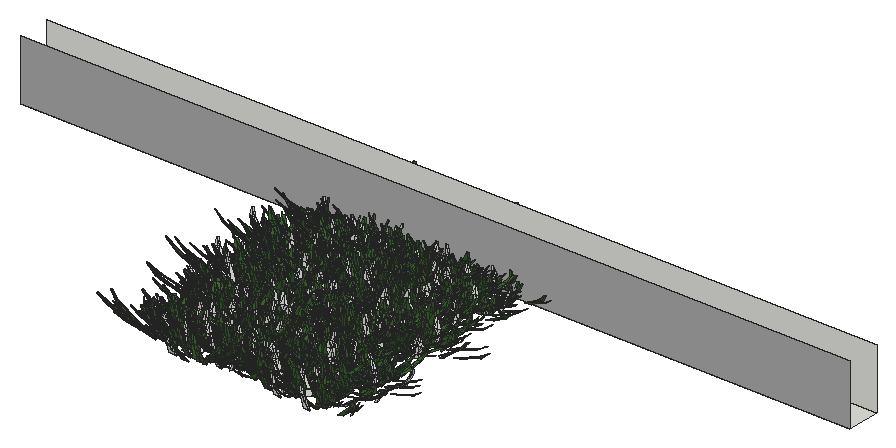
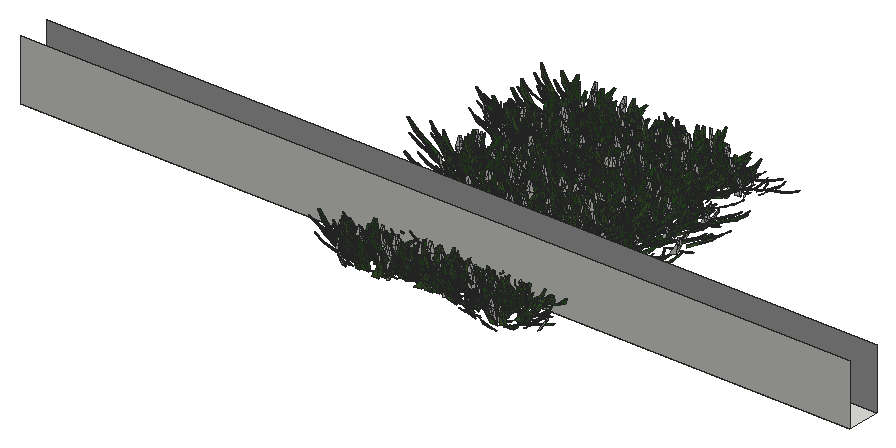
# SketchUp Ruby script. Lengths in inches.
U = 1.inch
M = Sketchup.active_model
def pt(a) = Geom::Point3d.new(a.map { |v| v * U })
def face(e, loops, mat)
  f = e.add_face(loops[0].map { |a| pt(a) })
  loops[1..].each { |l| e.add_face(l.map { |a| pt(a) }).erase! }
  f.material = f.back_material = mat if mat
  f
end
# faces: each face lists its corners as indices into pts; further lists are holes
def faces(e, pts, list, mat = nil) = list.each { |f| face(e, (f[0].is_a?(Array) ? f : [f]).map { |l| l.map { |i| pts[i] } }, mat) }
# xy, xz, yz: faces in a plane at the given z, y or x. An outline is a flat list of corners, or four numbers for a rectangle; further outlines are holes
def ring(l) = l.size == 4 ? [[l[0], l[1]], [l[2], l[1]], [l[2], l[3]], [l[0], l[3]]] : l.each_slice(2).to_a
def flat(e, list, mat, &to3) = list.each { |f| face(e, (f[0].is_a?(Array) ? f : [f]).map { |l| ring(l).map { |u, v| to3.(u, v) } }, mat) }
def xy(e, z, list, mat = nil) = flat(e, list, mat) { |x, y| [x, y, z] }
def xz(e, y, list, mat = nil) = flat(e, list, mat) { |x, z| [x, y, z] }
def yz(e, x, list, mat = nil) = flat(e, list, mat) { |y, z| [x, y, z] }
def lines(e, pts, list) = list.each { |a, b| e.add_line(pt(pts[a]), pt(pts[b])) }
# prism: a flat outline (further loops are holes) pulled along v
def prism(e, loops, v, mat = nil)
  f = face(e, loops, mat); d = Geom::Vector3d.new(v.map { |x| x * U })
  f.pushpull(f.normal.samedirection?(d) ? d.length : -d.length)
end
def box(e, o, s, mat = nil) = prism(e, [[o, [o[0] + s[0], o[1], o[2]], [o[0] + s[0], o[1] + s[1], o[2]], [o[0], o[1] + s[1], o[2]]]], [0, 0, s[2]], mat)
def at(x, y, z, deg = 0) = Geom::Transformation.translation(pt([x, y, z])) * Geom::Transformation.rotation(ORIGIN, Z_AXIS, deg.degrees)
def axes(o, x, y, z) = Geom::Transformation.new([*x, 0, *y, 0, *z, 0, *pt(o).to_a, 1])
def part(name) = M.definitions.add(name)
# library, detail: a bought-in or finely detailed component or shape, given as its bounding box
def library(name, o, s) = part(name).tap { |d| box(d.entities, o, s) }
def detail(e, o, s) = box(e.add_group.entities, o, s)
def put(e, d, t, mat = nil) = e.add_instance(d, t).tap { |i| i.material = mat if mat }
def group(e, t, mat = nil) = e.add_group.tap { |g| g.transformation = t; g.material = mat if mat }.entities
root = M.entities
M.materials.add("Material82").color = [68, 110, 58]
M.materials.add("Material83").color = [48, 90, 38]
M.materials.add("Material84").color = [68, 110, 48]
M.materials.add("Material85").color = [48, 90, 48]
M.materials.add("Material86").color = [58, 110, 58]
M.materials.add("Material87").color = [58, 90, 38]
M.materials.add("Material88").color = [68, 100, 58]
M.materials.add("Material89").color = [48, 100, 38]
M.materials.add("[Color M03]1").color = [170, 170, 170]
c1 = part("grass00")
p = [[-0.6875,0.15,0],[-0.56,0.08,5.52],[-0.04,0.03,2.76],[0.48,-0.02,0],[0.35,-0.02,5.52],[-0.1,-0.14,5.52],
  [-0.12,0.65,8.37],[-0.42,0.65,8.37]]
faces(c1.entities,p,[[0,1,2,3],[3,2,4],[1,5,2],[5,4,2],[1,6,5],[4,5,6],[7,6,1]])
c2 = part("Group16\#1")
put(c2.entities,c1,axes([1.44,-0.61,-0.01],[0.05352,0.12609,0],[-0.10704,0.04543,0.07239],[0.06664,-0.02828,0.11628]),"Material85")
put(c2.entities,c1,axes([0.76,-0.15,-0.01],[0.04676,0.24062,0],[-0.23162,0.04501,0.06642],[0.0652,-0.01267,0.23595]),"Material82")
put(c2.entities,c1,axes([0.79,0.01,-0.01],[-0.00606,0.34651,0],[-0.34381,-0.00602,0.0432],[0.04319,0.00076,0.34386]))
put(c2.entities,c1,axes([1,0.23,-0.01],[-0.07192,0.31144,0],[-0.28722,-0.06632,0.1236],[0.12043,0.02781,0.29478]),"Material84")
put(c2.entities,c1,axes([1.66,0.77,-0.01],[-0.13828,0.29651,0],[-0.21551,-0.1005,0.22471],[0.20365,0.09498,0.23779]),"Material89")
put(c2.entities,c1,axes([0.6875,0.52,-0.01],[-0.18126,0.24051,0],[-0.22746,-0.17142,0.09788],[0.07817,0.05891,0.28481]),"Material84")
put(c2.entities,c1,axes([0.68,0.78,-0.01],[-0.215,0.18688,0],[-0.12385,-0.14248,0.21334],[0.13995,0.16101,0.18878]),"Material82")
put(c2.entities,c1,axes([0.56,1,-0.01],[-0.13756,0.07624,0],[-0.06159,-0.11112,0.0927],[0.04494,0.08108,0.12705]),"Material84")
put(c2.entities,c1,axes([0.2,0.64,-0.01],[-0.23729,0.07254,0],[-0.05711,-0.18681,0.153],[0.04473,0.14632,0.19535]),"Material89")
put(c2.entities,c1,axes([0.0625,0.72,-0.01],[-0.28874,0.02525,0],[-0.02179,-0.24916,0.14647],[0.01276,0.14591,0.25012]),"Material82")
put(c2.entities,c1,axes([-0.08,0.62,-0.01],[-0.34089,-0.04187,0],[0.03255,-0.26504,0.216],[-0.02633,0.21439,0.26703]),"Material89")
put(c2.entities,c1,axes([-0.34,0.98,-0.01],[-0.14314,-0.0493,0],[0.04397,-0.12769,0.06843],[-0.02228,0.0647,0.13505]),"Material89")
put(c2.entities,c1,axes([-0.87,1.45,-0.01],[-0.23488,-0.14114,0],[0.13761,-0.22901,0.06087],[-0.03135,0.05217,0.26717]))
put(c2.entities,c1,axes([-0.72,0.77,-0.01],[-0.14208,-0.13251,0],[0.07209,-0.0773,0.16301],[-0.11118,0.11922,0.1057]),"Material89")
put(c2.entities,c1,axes([-0.62,0.43,-0.01],[-0.14845,-0.21203,0],[0.18654,-0.13061,0.12304],[-0.10079,0.07057,0.22772]),"Material82")
put(c2.entities,c1,axes([-0.68,0.29,-0.01],[-0.13639,-0.32136,0],[0.31723,-0.13464,0.05579],[-0.05136,0.0218,0.34462]),"Material83")
put(c2.entities,c1,axes([-0.64,0.125,-0.01],[-0.0458,-0.23569,0],[0.22124,-0.043,0.08276],[-0.08124,0.01579,0.22538]),"Material86")
put(c2.entities,c1,axes([-1.6,-0.03,-0.01],[0.00576,-0.32897,0],[0.27526,0.00482,0.18018],[-0.18015,-0.00315,0.2753]),"Material84")
put(c2.entities,c1,axes([-1.36,-0.31,-0.01],[0.05718,-0.24765,0],[0.18172,0.04196,0.17267],[-0.16825,-0.03885,0.1865]),"Material89")
put(c2.entities,c1,axes([-1.54,-0.72,-0.01],[0.06537,-0.14017,0],[0.13555,0.06321,0.03939],[-0.0357,-0.01665,0.14956]))
put(c2.entities,c1,axes([-1.19,-0.9,-0.01],[0.09597,-0.12735,0],[0.11214,0.08451,0.07557],[-0.06035,-0.04548,0.14042]),"Material88")
put(c2.entities,c1,axes([-0.47,-0.54,-0.01],[0.11588,-0.10072,0],[0.0618,0.0711,0.12124],[-0.07953,-0.0915,0.0942]))
put(c2.entities,c1,axes([-0.47,-0.84,-0.01],[0.11927,-0.0661,0],[0.06603,0.11913,0.00646],[-0.00313,-0.00565,0.13621]),"Material84")
put(c2.entities,c1,axes([-0.38,-1.24,-0.01],[0.28037,-0.08571,0],[0.0618,0.20215,0.20315],[-0.05939,-0.19428,0.21139]),"Material88")
put(c2.entities,c1,axes([-0.06,-0.66,-0.01],[0.22719,-0.01987,0],[0.01247,0.14255,0.17758],[-0.01547,-0.17691,0.1431]),"Material87")
put(c2.entities,c1,axes([0.11,-0.89,-0.01],[0.14882,0.01828,0],[-0.01058,0.08611,0.12229],[0.01491,-0.12138,0.08676]),"Material85")
put(c2.entities,c1,axes([0.25,-0.72,-0.01],[0.20481,0.07053,0],[-0.06206,0.18022,0.10291],[0.03351,-0.0973,0.1906]),"Material85")
put(c2.entities,c1,axes([0.85,-1.42,-0.01],[0.16481,0.09904,0],[-0.09472,0.15762,0.05616],[0.02893,-0.04814,0.18389]),"Material84")
put(c2.entities,c1,axes([1.01,-1.09,-0.01],[0.21858,0.20385,0],[-0.17495,0.1876,0.15339],[0.10462,-0.11218,0.25652]),"Material89")
put(c2.entities,c1,axes([1.01,-0.71,-0.01],[0.08733,0.12473,0],[-0.06445,0.04512,0.13037],[0.1068,-0.07477,0.07867]),"Material85")
c3 = part("Group15\#1")
put(c3.entities,c2,at(0,0,0))
c4 = part("3darcstudiotree_grass00\#1")
put(c4.entities,c3,at(0,0,0))
xy(root,-29.74,[[626.34,1040.81,782.4375,1046.93]])
xz(root,1040.81,[[626.34,-29.74,782.4375,-18.36]],"[Color M03]1")
xz(root,1046.93,[[626.34,-29.74,782.4375,-18.36]])
put(root,c4,axes([685.26,1045.64,-29.74],[3.16719,1.22877,0],[-2.37702,0.9529,-0.00671],[-0.02839,0.01138,1.53359]))
put(root,c4,axes([685.24,1030.39,-29.74],[3.90875,0.99817,0],[-2.33451,1.4218,-0.02279],[-0.07245,0.04412,1.88252]))
put(root,c4,axes([685.8125,1020.67,-29.74],[4.17909,0.84834,0],[-2.02565,1.55199,-0.04224],[-0.09233,0.07074,1.58426]))
put(root,c4,axes([686.23,1000.44,-29.74],[3.56991,0.07978,0],[-0.21949,1.52742,-0.02759],[-0.00848,0.05902,1.57942]))
put(root,c4,axes([686.15,1053.28,-29.74],[1.29207,1.70529,0],[-3.1938,0.37636,-0.01522],[-0.08109,0.00956,1.38916]))
put(root,c4,axes([688.03,1013.6,-29.74],[-4.32084,-0.18562,0],[0.42888,-1.55273,-0.0047],[0.00255,-0.00922,1.4854]))
put(root,c4,axes([686.48,1027.98,-29.74],[0.16976,1.81896,0],[-4.60297,0.06681,-0.03073],[-0.13236,0.00192,1.48809]))
put(root,c4,axes([688.1,1042.1,-29.74],[-3.93222,-0.02635,0],[0.07503,-1.74154,-0.03595],[0.00307,-0.07126,1.66434]))
put(root,c4,axes([688.4,1030.11,-29.74],[-3.5417,-0.59044,0],[1.62012,-1.51145,-0.0473],[0.08471,-0.07903,1.43445]))
put(root,c4,axes([686.59,1012.4,-29.74],[4.0668,0.76332,0],[-1.54133,1.27718,-0.01473],[-0.03515,0.02913,1.49308]))
put(root,c4,axes([688.18,1016.9,-29.74],[-3.98791,0.79031,0],[-1.65069,-1.29546,-0.0516],[-0.1637,-0.12847,1.94674]))
put(root,c4,axes([688.71,1020.82,-29.74],[-3.83726,0.13979,0],[-0.31883,-1.36117,-0.04806],[-0.027,-0.11528,1.58689]))
put(root,c4,axes([688.46,1039.78,-29.74],[2.03121,-1.05332,0],[3.7313,1.11909,-0.04371],[0.13933,0.04179,1.40723]))
put(root,c4,axes([689.43,1049.32,-29.74],[-3.73597,-0.76469,0],[1.79369,-1.36294,-0.02416],[0.05526,-0.04199,1.4491]))
put(root,c4,axes([689.48,1046.82,-29.74],[-2.98813,-0.54786,0],[1.47052,-1.24742,-0.04575],[0.11826,-0.10032,1.60296]))
put(root,c4,axes([688.39,1034.5,-29.74],[1.22817,1.22832,0],[-3.29828,0.51292,-0.04901],[-0.28268,0.04396,1.64754]))
put(root,c4,axes([689.55,1009.17,-29.74],[-3.41944,0.15794,0],[-0.40533,-1.36487,-0.03745],[-0.0251,-0.08453,1.50509]))
put(root,c4,axes([688.25,1003.46,-29.74],[0.51016,1.70246,0],[-4.00788,0.18679,-0.00527],[-0.02601,0.00121,1.50433]))
put(root,c4,axes([688.85,1052.03,-29.74],[3.58477,-0.09461,0],[0.24683,1.45461,-0.02393],[0.00869,0.05119,1.50627]))
put(root,c4,axes([688.72,1031.39,-29.74],[3.76255,0.21279,0],[-0.50611,1.39184,-0.02285],[-0.01632,0.04489,1.34478]))
put(root,c4,axes([690.19,999.18,-29.74],[-4.15336,0.88478,0],[-2.07336,-1.51373,-0.03525],[-0.06704,-0.04895,1.3087]))
put(root,c4,axes([690.36,1006.1,-29.74],[1.23783,-1.57966,0],[3.18362,0.388,-0.00928],[0.06663,0.00812,1.87692]))
put(root,c4,axes([689.19,1018.83,-29.74],[4.18297,0.824,0],[-1.87304,1.47883,-0.04234],[-0.08644,0.06825,1.4356]))
put(root,c4,axes([689.72,1038.62,-29.74],[3.73542,0.56333,0],[-1.36375,1.40645,-0.02441],[-0.06005,0.06193,1.97124]))
put(root,c4,axes([689.6875,1036.05,-29.74],[4.26727,0.66803,0],[-1.41698,1.40776,-0.04113],[-0.07249,0.07202,1.37498]))
put(root,c4,axes([690.2,1044.36,-29.74],[1.59793,1.26945,0],[-3.48077,0.68144,-0.01001],[-0.04528,0.00886,1.4706]))
put(root,c4,axes([692.05,1026.61,-29.74],[-4.24589,-0.20577,0],[0.52914,-1.69815,-0.04768],[0.02678,-0.08595,1.49744]))
put(root,c4,axes([690.56,1011.83,-29.74],[0.88024,1.52698,0],[-4.39329,0.39388,-0.06457],[-0.26955,0.02417,1.44574]))
put(root,c4,axes([691.59,1001.02,-29.74],[2.74133,-1.23391,0],[3.31507,1.14547,-0.04981],[0.18948,0.06547,1.67091]))
put(root,c4,axes([690.7,1024.72,-29.74],[3.13752,1.05459,0],[-2.29496,1.06192,-0.00613],[-0.02513,0.01163,1.67562]))
put(root,c4,axes([691.56,1006.93,-29.74],[1.5924,1.20755,0],[-3.44476,0.70651,-0.03549],[-0.1652,0.03388,1.52707]))
put(root,c4,axes([691.34,1023.18,-29.74],[1.54833,1.52017,0],[-4.09421,0.64856,-0.00669],[-0.03642,0.00577,1.94122]))
put(root,c4,axes([694.31,998.22,-29.74],[-1.94812,-1.05267,0],[3.13916,-0.90354,-0.00015],[0.00082,-0.00024,1.94435]))
put(root,c4,axes([694.01,1022.625,-29.74],[-0.04856,-1.33378,0],[4.56796,-0.02587,-0.06189],[0.3016,-0.00171,1.66883]))
put(root,c4,axes([694.35,1049.73,-29.74],[-2.95598,-0.91326,0],[2.43781,-1.22721,-0.04081],[0.12436,-0.0626,1.46417]))
put(root,c4,axes([694.3,1040.13,-29.74],[-3.68784,-0.24252,0],[0.55953,-1.32329,-0.01602],[0.01459,-0.0345,1.41148]))
put(root,c4,axes([694.9,1051.66,-29.74],[-0.4279,-1.35562,0],[4.45161,-0.21854,-0.05859],[0.31746,-0.01559,1.83593]))
put(root,c4,axes([695.24,1029.53,-29.74],[-4.54384,0.18076,0],[-0.35947,-1.40543,-0.00469],[-0.00344,-0.01343,1.96044]))
put(root,c4,axes([695.49,1031.91,-29.74],[-3.59063,0.36551,0],[-0.927,-1.41632,-0.03018],[-0.05381,-0.08221,1.98332]))
put(root,c4,axes([696,1046.29,-29.74],[-3.48173,-0.56284,0],[1.61416,-1.55298,-0.01809],[0.03189,-0.03068,1.4829]))
put(root,c4,axes([695.47,1044.32,-29.74],[1.06749,-1.46896,0],[3.76494,0.42553,-0.03571],[0.22932,0.02592,1.9611]))
put(root,c4,axes([695.58,1001.4,-29.74],[-3.26554,0.66263,0],[-1.53451,-1.17616,-0.01759],[-0.06154,-0.04717,1.92222]))
put(root,c4,axes([695.37,1013.97,-29.74],[2.51439,-1.31879,0],[3.78,1.12088,-0.05965],[0.2657,0.07879,1.97549]))
put(root,c4,axes([694.59,1036.05,-29.74],[4.03419,0.29669,0],[-0.75311,1.59264,-0.00417],[-0.00465,0.00984,1.87295]))
put(root,c4,axes([696.16,1015.69,-29.74],[-0.70547,-1.57622,0],[3.40493,-0.23702,-0.01992],[0.12135,-0.00845,1.60321]))
put(root,c4,axes([694.59,1009.8,-29.74],[4.47557,0.19067,0],[-0.50576,1.84642,-0.03307],[-0.01603,0.05854,1.59331]))
put(root,c4,axes([695.01,1025.3,-29.74],[0.58274,1.76141,0],[-3.38049,0.17394,-0.03746],[-0.24477,0.01259,1.68385]))
put(root,c4,axes([695.69,1007,-29.74],[-3.09447,0.74267,0],[-2.17746,-1.41107,-0.01391],[-0.03982,-0.0258,1.7292]))
put(root,c4,axes([695.91,1011.56,-29.74],[2.464,-1.39681,0],[2.85004,0.78193,-0.02795],[0.16419,0.04505,1.86246]))
put(root,c4,axes([695.58,1033.86,-29.74],[-1.9685,1.46825,0],[-4.07305,-0.84931,-0.01892],[-0.07094,-0.01479,1.46501]))
put(root,c4,axes([697.32,1042.58,-29.74],[-2.90199,-1.04001,0],[2.97522,-1.29119,-0.02206],[0.0727,-0.03155,1.62457]))
put(root,c4,axes([695.81,1019.07,-29.74],[-1.84293,1.54258,0],[-3.69335,-0.68627,-0.00165],[-0.00726,-0.00135,1.48801]))
put(root,c4,axes([697.4,1002.77,-29.74],[-4.60496,-0.17881,0],[0.42059,-1.68464,-0.00134],[0.00055,-0.00219,1.33719]))
put(root,c4,axes([695.52,1038.96,-29.74],[1.66114,1.62878,0],[-3.87747,0.61504,-0.0015],[-0.00686,0.00109,1.54039]))
put(root,c4,axes([696.98,1005.53,-29.74],[2.67997,-1.42027,0],[3.59345,1.05458,-0.05496],[0.18586,0.05455,1.41537]))
put(root,c4,axes([697.18,1020.51,-29.74],[0.63899,1.37464,0],[-4.27438,0.30902,-0.00804],[-0.04314,0.00312,1.77733]))
put(root,c4,axes([697.42,1027.89,-29.74],[1.87438,1.56788,0],[-3.52749,0.65588,-0.03917],[-0.21764,0.04047,1.79585]))
put(root,c4,axes([699.9375,1003.08,-29.74],[-1.02752,-1.39563,0],[3.42384,-0.39205,-0.00444],[0.02976,-0.00341,1.86591]))
put(root,c4,axes([699.36,1022.7,-29.74],[1.33366,-1.36849,0],[3.54112,0.53673,-0.03841],[0.22056,0.03343,1.74904]))
put(root,c4,axes([699.84,1031.28,-29.74],[-1.96103,-1.06216,0],[3.43549,-0.98649,-0.06067],[0.27868,-0.08002,1.80988]))
put(root,c4,axes([699.73,1007.51,-29.74],[-3.04968,0.59415,0],[-1.75652,-1.40223,-0.03032],[-0.06781,-0.05413,1.50108]))
put(root,c4,axes([699.7,1038.84,-29.74],[3.38929,-0.88137,0],[2.3631,1.41334,-0.02666],[0.06787,0.04059,1.48784]))
put(root,c4,axes([700.71,1051.15,-29.74],[0.25727,-1.4604,0],[3.98489,0.10918,-0.0172],[0.09613,0.00263,1.67763]))
put(root,c4,axes([700.31,999.79,-29.74],[-2.6125,1.23987,0],[-2.75746,-0.90365,-0.04997],[-0.20997,-0.06881,1.46822]))
put(root,c4,axes([701.4,1036.89,-29.74],[-3.77025,-0.95024,0],[2.35793,-1.45505,-0.05584],[0.17762,-0.10961,1.93872]))
put(root,c4,axes([700.04,1006.09,-29.74],[-0.25979,1.36498,0],[-3.68566,-0.1091,-0.02554],[-0.15097,-0.00447,1.64241]))
put(root,c4,axes([701.8,1011.36,-29.74],[-4.34871,0.30764,0],[-0.79873,-1.75601,-0.00093],[-0.00077,-0.00169,1.58752]))
put(root,c4,axes([700.61,1001.57,-29.74],[3.80887,0.06416,0],[-0.18164,1.67717,-0.01987],[-0.00391,0.03608,1.47043]))
put(root,c4,axes([700.63,1014.125,-29.74],[4.17174,-0.07865,0],[0.15922,1.3134,-0.03217],[0.01066,0.0879,1.73328]))
put(root,c4,axes([700.83,1016.18,-29.74],[3.86863,-0.34225,0],[0.73265,1.28801,-0.00297],[0.00437,0.00768,1.68702]))
put(root,c4,axes([702.52,1046.97,-29.74],[-2.85085,-0.66888,0],[2.41654,-1.60188,-0.00321],[0.00686,-0.00455,1.48019]))
put(root,c4,axes([701.73,1039.84,-29.74],[-3.53825,1.08299,0],[-2.59336,-1.31776,-0.03049],[-0.10241,-0.05204,1.73706]))
put(root,c4,axes([701.04,1025.99,-29.74],[3.26947,0.70015,0],[-1.66816,1.21153,-0.03457],[-0.12105,0.08791,1.92264]))
put(root,c4,axes([702,1045.13,-29.74],[2.00503,-1.14609,0],[3.00042,0.81639,-0.0362],[0.21042,0.05725,1.92943]))
put(root,c4,axes([701.6,1010.31,-29.74],[-1.46805,1.46647,0],[-4.14161,-0.64484,-0.02576],[-0.10998,-0.01712,1.53201]))
put(root,c4,axes([701.68,1018.24,-29.74],[4.25624,-0.01859,0],[0.03959,1.4097,-0.01976],[0.00112,0.03979,1.36845]))
put(root,c4,axes([701.92,1029.43,-29.74],[2.49415,0.97261,0],[-2.31115,0.92177,-0.02576],[-0.13853,0.05525,1.88472]))
put(root,c4,axes([702.02,1033.34,-29.74],[4.40385,0.48107,0],[-1.25638,1.78876,-0.02222],[-0.03253,0.04631,1.93436]))
put(root,c4,axes([702.35,1049.27,-29.74],[2.4354,1.06288,0],[-2.86607,1.02137,-0.0306],[-0.14622,0.05211,1.86488]))
put(root,c4,axes([703.14,1020.0625,-29.74],[-2.30622,1.23379,0],[-2.8482,-0.82802,-0.0238],[-0.11552,-0.03358,1.59896]))
put(root,c4,axes([702.49,1043.29,-29.74],[1.42863,1.44478,0],[-4.37041,0.67213,-0.01645],[-0.07678,0.01181,1.76201]))
put(root,c4,axes([702.76,1028.11,-29.74],[1.30118,1.34593,0],[-3.49846,0.52602,-0.01397],[-0.0708,0.01064,1.52193]))
put(root,c4,axes([705.33,1001.875,-29.74],[-2.87014,-1.48867,0],[3.23188,-0.96911,-0.02],[0.09309,-0.02792,1.779]))
put(root,c4,axes([705.11,1003.27,-29.74],[-0.3493,-1.81077,0],[4.63308,-0.139,-0.05882],[0.26935,-0.00808,1.5994]))
put(root,c4,axes([705.48,1014.95,-29.74],[-3.58056,-0.39826,0],[0.95821,-1.33984,-0.015],[0.02011,-0.02812,1.30652]))
put(root,c4,axes([704.68,1047.25,-29.74],[-0.87127,1.65753,0],[-3.69619,-0.30217,-0.02464],[-0.15319,-0.01252,1.79662]))
put(root,c4,axes([705.34,1005.5625,-29.74],[-3.11874,1.35551,0],[-2.91461,-1.04296,-0.0082],[-0.03562,-0.01275,1.73071]))
put(root,c4,axes([705.0625,1045.39,-29.74],[-0.23965,1.40351,0],[-3.9598,-0.10516,-0.04305],[-0.25813,-0.00685,1.78778]))
put(root,c4,axes([706.1,1028.82,-29.74],[-4.32286,0.64319,0],[-1.64772,-1.72238,-0.03096],[-0.05617,-0.05872,1.79846]))
put(root,c4,axes([706.66,1012.73,-29.74],[-3.23633,-0.50825,0],[1.72306,-1.70642,-0.01803],[0.03469,-0.03435,1.81493]))
put(root,c4,axes([705.58,1024.93,-29.74],[-1.77081,1.15286,0],[-3.98211,-0.9513,-0.05645],[-0.27396,-0.06545,1.97994]))
put(root,c4,axes([706.92,1041.2,-29.74],[-1.58728,-1.19948,0],[3.58979,-0.73882,-0.00435],[0.01908,-0.00393,1.50222]))
put(root,c4,axes([705.43,1023.25,-29.74],[2.97915,0.86965,0],[-2.38175,1.26898,-0.05487],[-0.15774,0.08404,1.44987]))
put(root,c4,axes([705.53,1049.07,-29.74],[0.67536,1.71011,0],[-3.33591,0.2049,-0.00889],[-0.04851,0.00298,1.39664]))
put(root,c4,axes([706.3125,1051.69,-29.74],[2.58879,-1.26718,0],[2.80569,0.89147,-0.02709],[0.14156,0.04498,1.8123]))
put(root,c4,axes([705.43,1036.52,-29.74],[3.8564,0.72862,0],[-1.8534,1.52567,-0.04599],[-0.08438,0.06946,1.36526]))
put(root,c4,axes([707.49,1042.22,-29.74],[-3.19208,-0.59663,0],[1.68588,-1.40285,-0.03887],[0.08271,-0.06882,1.46596]))
put(root,c4,axes([706.66,1021.08,-29.74],[3.36447,-1.00796,0],[2.1967,1.14039,-0.03309],[0.10605,0.05506,1.44206]))
put(root,c4,axes([707.93,1031.47,-29.74],[-2.97002,-0.61033,0],[1.81963,-1.37718,-0.0201],[0.04091,-0.03096,1.30027]))
put(root,c4,axes([708.11,1009.7,-29.74],[-3.57677,-1.09741,0],[2.84767,-1.44352,-0.06227],[0.15089,-0.07649,1.37168]))
put(root,c4,axes([706.35,1038.09,-29.74],[1.39303,1.55232,0],[-3.39855,0.47433,-0.0171],[-0.11021,0.01538,1.84743]))
put(root,c4,axes([706.98,999.38,-29.74],[-0.9025,1.72738,0],[-3.54084,-0.28772,-0.03296],[-0.16809,-0.01366,1.411]))
put(root,c4,axes([707.13,1018.53,-29.74],[-1.59741,1.49736,0],[-3.22806,-0.5356,-0.02216],[-0.12937,-0.02146,1.66252]))
put(root,c4,axes([708.16,1033.23,-29.74],[3.05945,-1.08948,0],[2.66485,1.16389,-0.04418],[0.16678,0.07284,1.67893]))
put(root,c4,axes([707.92,1007.3,-29.74],[-0.7508,1.54691,0],[-4.43091,-0.33447,-0.01652],[-0.07223,-0.00545,1.50529]))
put(root,c4,axes([708.11,1027.29,-29.74],[4.00478,-0.12141,0],[0.32544,1.66956,-0.03486],[0.01415,0.07259,1.68524]))
put(root,c4,axes([708.51,1016.2,-29.74],[3.83024,1.03121,0],[-2.22146,1.2833,-0.02215],[-0.08012,0.04629,1.8946]))
put(root,c4,axes([710.36,1031.82,-29.74],[0.46065,-1.85098,0],[4.3401,0.16799,-0.05803],[0.23131,0.00895,1.30918]))
put(root,c4,axes([711.16,1036.35,-29.74],[-2.75759,-1.29294,0],[3.16062,-1.04842,-0.04595],[0.19898,-0.066,1.75181]))
put(root,c4,axes([710.6875,1038.98,-29.74],[2.18609,-1.17283,0],[3.5885,1.04029,-0.0227],[0.08817,0.02556,1.60931]))
put(root,c4,axes([711.4,1012.24,-29.74],[-3.68156,-0.36216,0],[0.87025,-1.37591,-0.04204],[0.06138,-0.09705,1.62585]))
put(root,c4,axes([711.06,998.85,-29.74],[-3.79448,1.12109,0],[-2.55555,-1.34526,-0.03017],[-0.0978,-0.05148,1.72726]))
put(root,c4,axes([710.34,1034.34,-29.74],[1.1355,1.36945,0],[-3.88951,0.50159,-0.05705],[-0.27012,0.03483,1.52794]))
put(root,c4,axes([712.04,1045.67,-29.74],[-3.52632,-0.01876,0],[0.05142,-1.50323,-0.03579],[0.00272,-0.07942,1.60809]))
put(root,c4,axes([711.43,1023.05,-29.74],[-3.10715,1.0196,0],[-2.89034,-1.36991,-0.01948],[-0.06651,-0.03152,1.80807]))
put(root,c4,axes([711.68,1052.16,-29.74],[-3.0378,0.91986,0],[-2.50548,-1.28689,-0.05552],[-0.17911,-0.092,1.63365]))
put(root,c4,axes([710.54,1041.97,-29.74],[1.49785,1.29889,0],[-3.32043,0.59552,-0.00419],[-0.02419,0.00434,1.73548]))
put(root,c4,axes([711.64,1020.54,-29.74],[3.31286,-0.55128,0],[1.80617,1.68812,-0.0407],[0.06877,0.06427,1.51351]))
put(root,c4,axes([710.9,1001.96,-29.74],[3.22227,0.82324,0],[-2.17222,1.32236,-0.01048],[-0.0296,0.01802,1.55517]))
put(root,c4,axes([713.05,1018.85,-29.74],[-4.269,-0.81813,0],[1.88917,-1.53314,-0.01545],[0.03796,-0.03081,1.8215]))
put(root,c4,axes([710.91,1046.58,-29.74],[2.65644,1.45338,0],[-3.09672,0.88031,-0.01552],[-0.06337,0.01801,1.43977]))
put(root,c4,axes([711.76,1014.21,-29.74],[0.15057,1.31453,0],[-3.70176,0.06595,-0.0329],[-0.23461,0.00418,1.98251]))
put(root,c4,axes([711.72,1006.3,-29.74],[-0.68682,1.71759,0],[-4.33467,-0.26958,-0.03641],[-0.15889,-0.00988,1.45326]))
put(root,c4,axes([711.82,1040.14,-29.74],[4.28771,-0.12133,0],[0.32919,1.80935,-0.01186],[0.00375,0.02059,1.52253]))
put(root,c4,axes([712.61,1052.92,-29.74],[2.17543,-1.37172,0],[2.92508,0.72149,-0.0272],[0.16226,0.04002,1.81972]))
put(root,c4,axes([712.15,1007.125,-29.74],[-1.33529,1.77622,0],[-3.16975,-0.37061,-0.00114],[-0.00828,-0.00097,1.86907]))
put(root,c4,axes([711.68,1015.79,-29.74],[1.34239,1.63135,0],[-4.02681,0.51535,-0.01715],[-0.07258,0.00929,1.41194]))
put(root,c4,axes([712.77,1025.18,-29.74],[-1.89402,1.2029,0],[-3.60721,-0.88336,-0.02009],[-0.09037,-0.02213,1.68525]))
put(root,c4,axes([713.58,1027.93,-29.74],[-1.08101,1.66314,0],[-4.29936,-0.43462,-0.05431],[-0.26643,-0.02693,1.6847]))
put(root,c4,axes([713.96,1049.39,-29.74],[-2.99935,1.42497,0],[-3.08029,-1.00838,-0.00469],[-0.01919,-0.00628,1.59556]))
put(root,c4,axes([713.45,1029.88,-29.74],[2.63123,0.92373,0],[-2.85346,1.26414,-0.03405],[-0.11674,0.05172,1.65877]))
put(root,c4,axes([713.71,1009.82,-29.74],[2.81192,0.87479,0],[-2.84329,1.42145,-0.06164],[-0.14998,0.07498,1.3518]))
put(root,c4,axes([714.05,1003.16,-29.74],[0.48103,1.53156,0],[-4.51259,0.22043,-0.03401],[-0.13914,0.0068,1.40523]))
put(root,c4,axes([716.15,1034.75,-29.74],[1.2731,-1.20941,0],[3.44603,0.56418,-0.03248],[0.17294,0.02831,1.61223]))
put(root,c4,axes([716.53,1020.05,-29.74],[-3.65599,0.07986,0],[-0.21877,-1.55768,-0.04105],[-0.01403,-0.0999,1.83253]))
put(root,c4,axes([715.71,1036.68,-29.74],[-0.67685,1.82709,0],[-3.63349,-0.20935,-0.03578],[-0.17247,-0.00994,1.34076]))
put(root,c4,axes([716.55,998.26,-29.74],[-3.15287,0.69435,0],[-1.94177,-1.37131,-0.05669],[-0.17259,-0.12189,1.86391]))
put(root,c4,axes([717.15,1009.83,-29.74],[-2.36391,-1.30666,0],[2.88424,-0.81154,-0.04134],[0.24623,-0.06928,1.943]))
put(root,c4,axes([716.42,1004.16,-29.74],[-2.91503,0.96344,0],[-2.99535,-1.40954,-0.01682],[-0.05566,-0.02619,1.80026]))
put(root,c4,axes([716.77,1042.3,-29.74],[-3.36658,1.12781,0],[-2.16506,-1.00516,-0.00331],[-0.01262,-0.00586,1.47415]))
put(root,c4,axes([717.22,1008.5,-29.74],[2.5477,-1.31265,0],[2.99582,0.90433,-0.00025],[0.00104,0.00031,1.45509]))
put(root,c4,axes([717.06,1022.9,-29.74],[2.84002,-1.42543,0],[3.17904,0.98511,-0.04001],[0.1906,0.05906,1.83572]))
